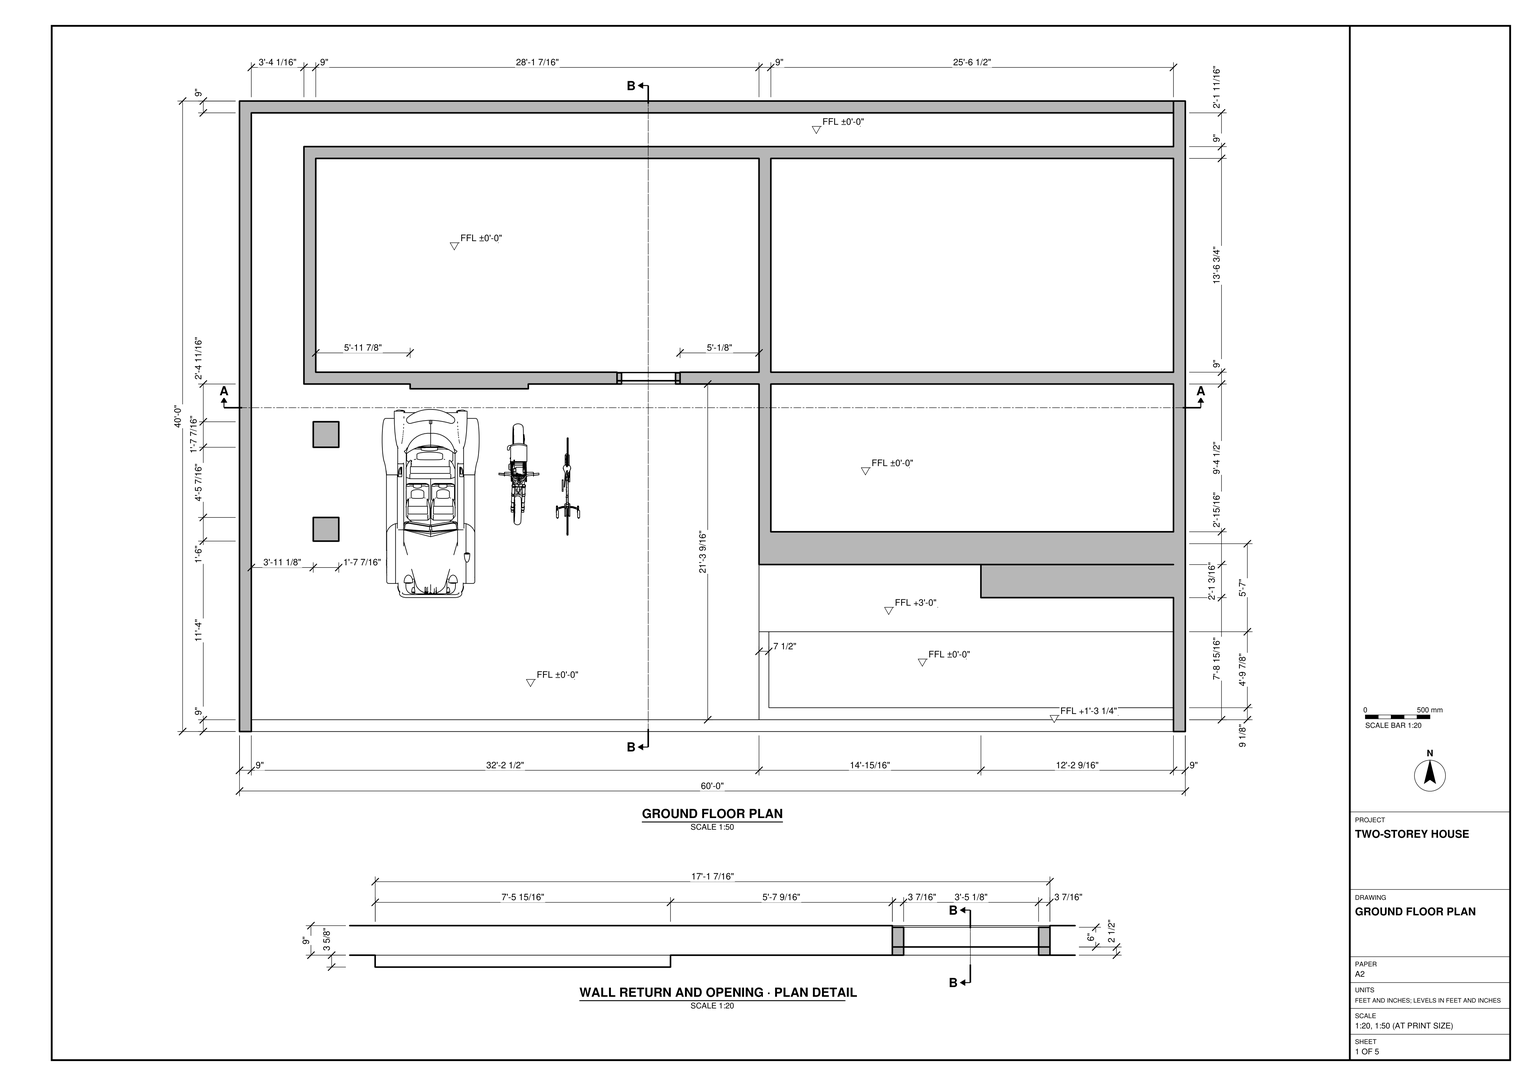
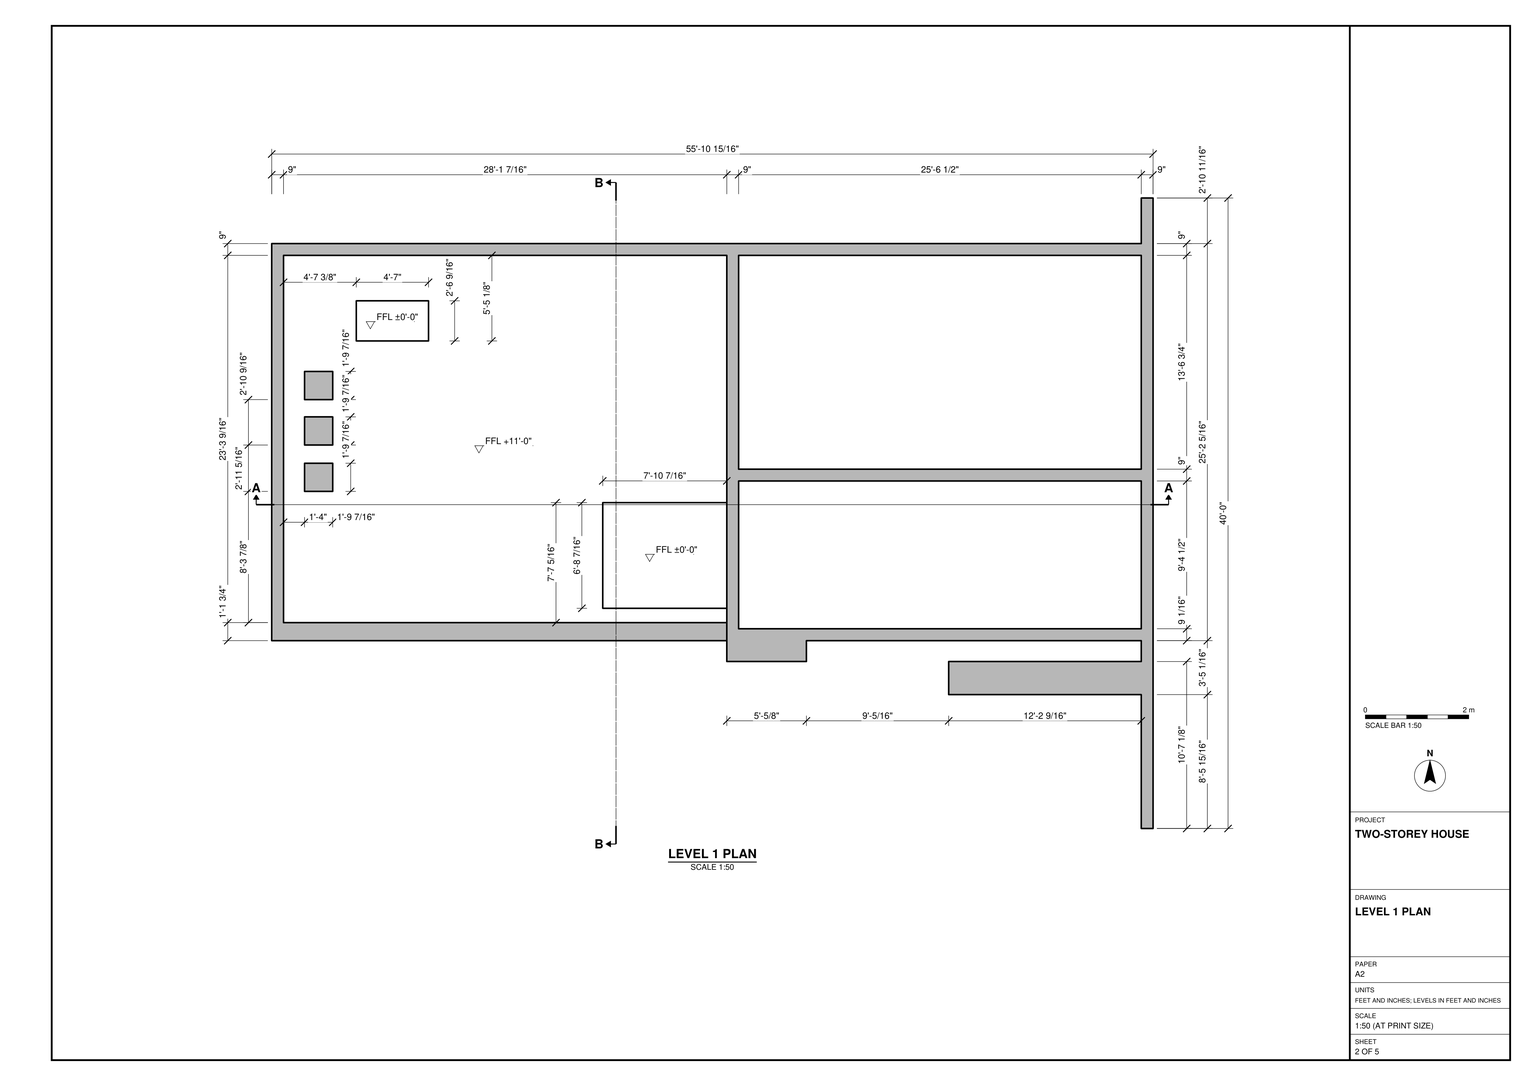
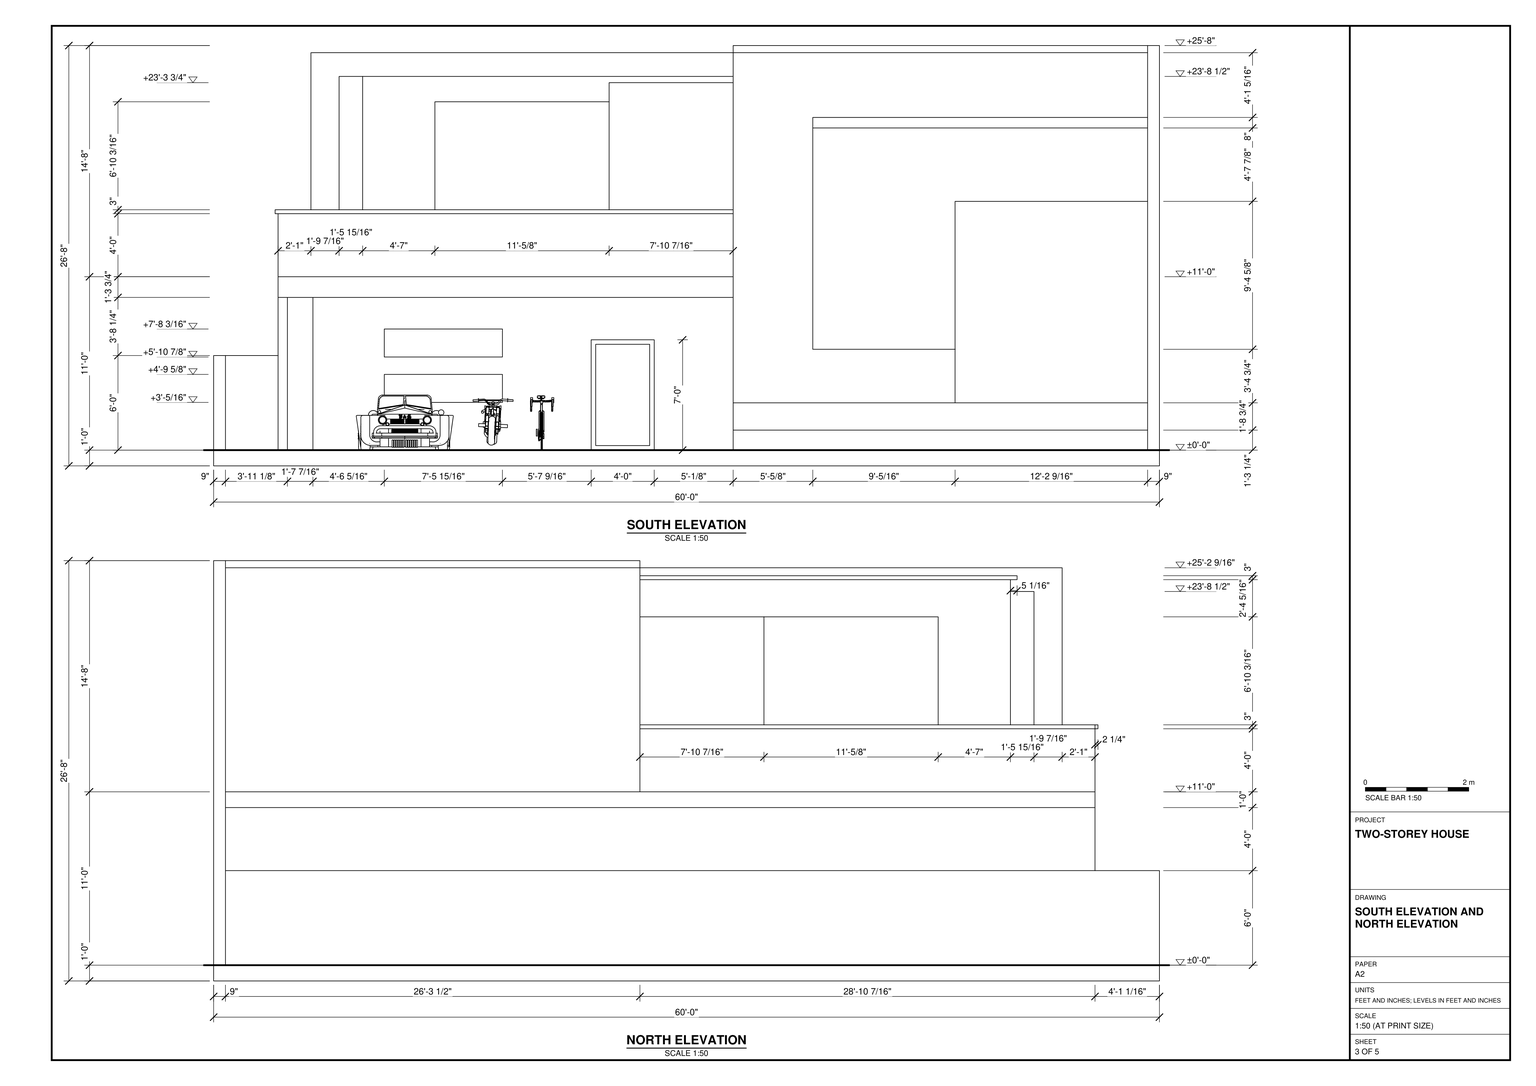
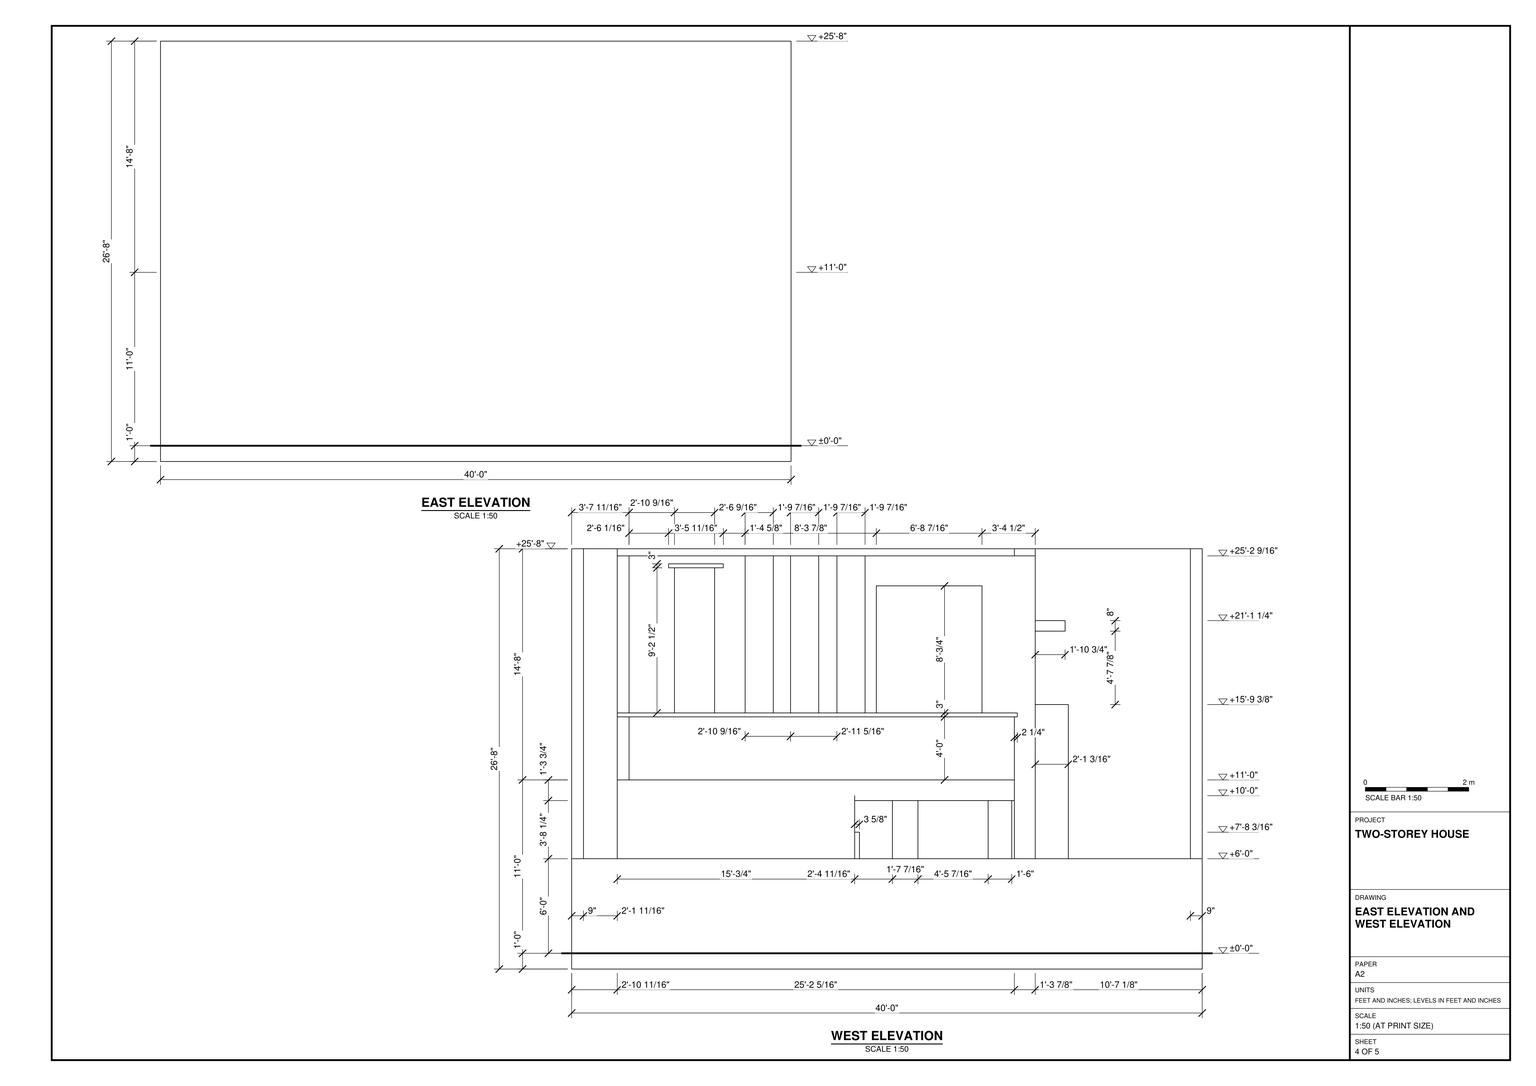
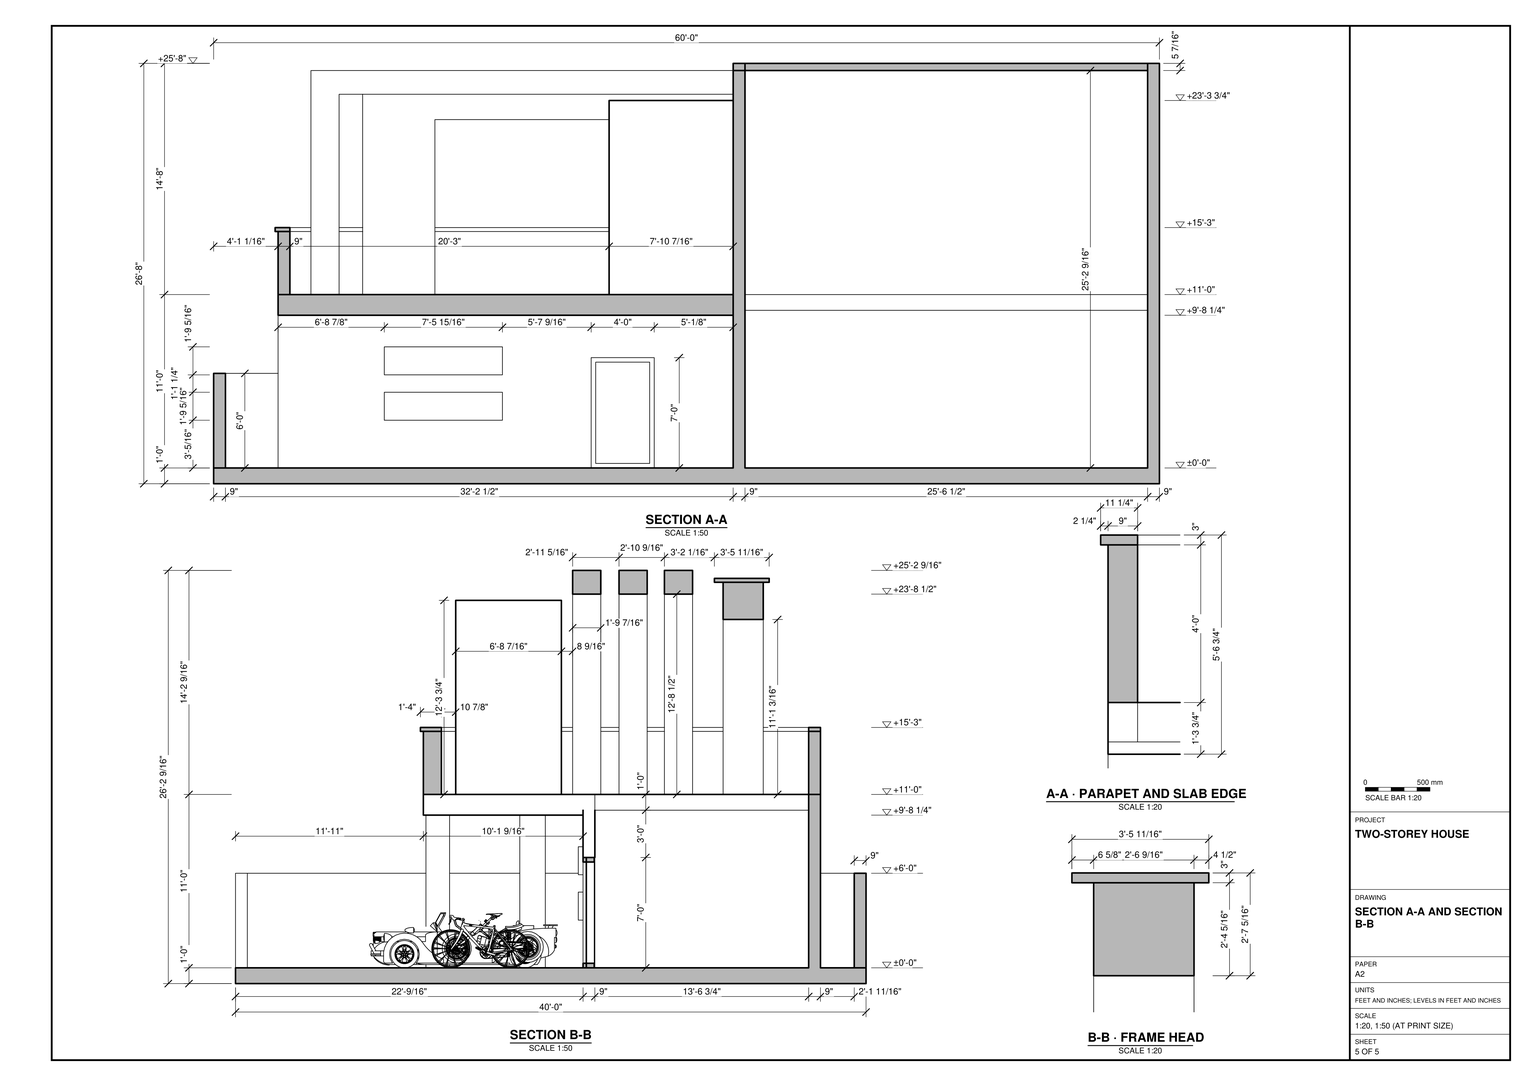
Build the house in SketchUp from task_files/diagram_01.pdf. Work in feet and inches. The overall model is 60'-0" wide from east to west, 40'-0" deep from north to south and 26'-8" high, including the base below the ground floor. Set the ground floor at ±0'-0" and the upper floor at +11'-0".

Use the plans to set out the perimeter walls, the enclosed rear bay and the divided east side of the house. Model the 9" walls with the thicker returns where drawn. Leave the parking bay open to the south, with the upper slab projecting over it and square supports along its west side. Place the car, motorcycle and bicycle as shown. Use the enlarged plan detail for the wall return and framed doorway behind the parking bay, and the south elevation for the window positions.

Carry the central dividing wall through the upper level. Match the slab edges, parapets and flat roof profiles to the elevations, including the tall rectangular frame on the east side of the south facade. Keep walls, slabs and roof elements separate, group each vehicle and any furniture or joinery piece separately, and use components for repeated parts. Decor and loose items may be any suitable library components. Save one SketchUp model as output_files/two_storey_house_with_a_covered_parking_bay.skp.

# SketchUp Ruby script. Lengths in inches.
U = 1.inch
M = Sketchup.active_model
def pt(a) = Geom::Point3d.new(a.map { |v| v * U })
def face(e, loops, mat)
  f = e.add_face(loops[0].map { |a| pt(a) })
  loops[1..].each { |l| e.add_face(l.map { |a| pt(a) }).erase! }
  f.material = f.back_material = mat if mat
  f
end
# faces: each face lists its corners as indices into pts; further lists are holes
def faces(e, pts, list, mat = nil) = list.each { |f| face(e, (f[0].is_a?(Array) ? f : [f]).map { |l| l.map { |i| pts[i] } }, mat) }
# xy, xz, yz: faces in a plane at the given z, y or x. An outline is a flat list of corners, or four numbers for a rectangle; further outlines are holes
def ring(l) = l.size == 4 ? [[l[0], l[1]], [l[2], l[1]], [l[2], l[3]], [l[0], l[3]]] : l.each_slice(2).to_a
def flat(e, list, mat, &to3) = list.each { |f| face(e, (f[0].is_a?(Array) ? f : [f]).map { |l| ring(l).map { |u, v| to3.(u, v) } }, mat) }
def xy(e, z, list, mat = nil) = flat(e, list, mat) { |x, y| [x, y, z] }
def xz(e, y, list, mat = nil) = flat(e, list, mat) { |x, z| [x, y, z] }
def yz(e, x, list, mat = nil) = flat(e, list, mat) { |y, z| [x, y, z] }
def lines(e, pts, list) = list.each { |a, b| e.add_line(pt(pts[a]), pt(pts[b])) }
# prism: a flat outline (further loops are holes) pulled along v
def prism(e, loops, v, mat = nil)
  f = face(e, loops, mat); d = Geom::Vector3d.new(v.map { |x| x * U })
  f.pushpull(f.normal.samedirection?(d) ? d.length : -d.length)
end
def box(e, o, s, mat = nil) = prism(e, [[o, [o[0] + s[0], o[1], o[2]], [o[0] + s[0], o[1] + s[1], o[2]], [o[0], o[1] + s[1], o[2]]]], [0, 0, s[2]], mat)
def at(x, y, z, deg = 0) = Geom::Transformation.translation(pt([x, y, z])) * Geom::Transformation.rotation(ORIGIN, Z_AXIS, deg.degrees)
def axes(o, x, y, z) = Geom::Transformation.new([*x, 0, *y, 0, *z, 0, *pt(o).to_a, 1])
def part(name) = M.definitions.add(name)
# library, detail: a bought-in or finely detailed component or shape, given as its bounding box
def library(name, o, s) = part(name).tap { |d| box(d.entities, o, s) }
def detail(e, o, s) = box(e.add_group.entities, o, s)
def put(e, d, t, mat = nil) = e.add_instance(d, t).tap { |i| i.material = mat if mat }
def group(e, t, mat = nil) = e.add_group.tap { |g| g.transformation = t; g.material = mat if mat }.entities
root = M.entities
M.materials.add("[Blinds Wood Natural]").color = [167, 145, 74]
M.materials.add("[Color B08]").color = [91, 37, 0]
M.materials.add("[Color D01]").color = [255, 242, 204]
M.materials.add("[Color E01]").color = [255, 255, 204]
M.materials.add("[Color M05]").color = [114, 114, 114]
M.materials.add("[Color M06]").color = [86, 86, 86]
M.materials.add("[Color_006]").color = [86, 86, 86]
M.materials.add("[Color_B02]").color = [255, 101, 50]
M.materials.add("[Granite Brown]").color = [126, 104, 91]
M.materials.add("[Grass Dark Green]").color = [106, 157, 55]
M.materials.add("[Metal Seamed]").color = [118, 119, 115]
M.materials.add("[Metal_Aluminum_Anodized]").color = [202, 209, 219]
M.materials.add("[Pavers with Grass Herringbone]").color = [197, 201, 190]
M.materials.add("[Translucent Glass Gray]").color = [128, 128, 128]
M.materials["[Translucent Glass Gray]"].alpha = 0.5
M.materials.add("[Translucent_Glass_Sky_Reflection]").color = [125, 138, 183]
M.materials["[Translucent_Glass_Sky_Reflection]"].alpha = 0.52
M.materials.add("[Wood Veneer 01]").color = [120, 70, 37]
M.materials.add("black1").color = [0, 0, 0]
c1 = library("Car body side",[-13.21,-32.42,-1.14],[59.58,225.6,51.3])
c2 = library("Car fender",[-16.61,0,0],[37.81,73.61,36.77])
c3 = library("Headlamp assembly",[0,0,0],[13.23,21.85,12.42])
c4 = part("Компонент\#2")
xy(c4.entities,0,[[0,2.9375,33.05,6.18]])
xy(c4.entities,23.57,[[4.41,9.77,33.05,11.46]],"[Color_B02]")
yz(c4.entities,0,[[0,0,0,5.92,7.73,19.89,9.03,19.17,1.69,5.92,6.18,0]],"[Color_B02]")
yz(c4.entities,1.28,[[1.01,6.8,6.85,17.36,6.45,17.58,0.61,7.02]],"[Color_006]")
yz(c4.entities,4.41,[[11.0625,22.85,9.77,23.57,11.46,23.57]],"[Color_B02]")
yz(c4.entities,31.57,[[3.7,11.67,3.3,11.89,9.17,22.49,9.5625,22.27]],"[Color_006]")
yz(c4.entities,33.05,[[2.9375,0,6.18,0,2.9375,4.28],[2.9375,4.28,1.69,5.92,2.9375,8.17]])
yz(c4.entities,33.05,[[2.9375,8.17,11.46,23.57,9.77,23.57,2.9375,11.23]],"[Color_006]")
p = [[0,0,0],[33.05,2.9375,11.23],[0,0,5.92],[3.91,0.35,2.11],[3.67,0.33,1.75],[3.34,0.3,1.46],
  [2.94,0.26,1.27],[2.52,0.22,1.1875],[2.08,0.18,1.22],[1.67,0.15,1.36],[1.31,0.12,1.61],[1.02,0.09,1.94],
  [0.83,0.07,2.34],[0.75,0.07,2.77],[0.78,0.07,3.2],[0.93,0.08,3.62],[1.17,0.1,3.98],[1.5,0.13,4.26],
  [1.9,0.17,4.45],[2.32,0.21,4.54],[2.76,0.25,4.5],[3.17,0.28,4.36],[3.53,0.3125,4.11],[3.82,0.34,3.78],
  [4.01,0.36,3.39],[4.09,0.36,2.96],[4.06,0.36,2.52],[0,6.18,0],[0,1.69,5.92],[33.05,1.69,5.92],
  [33.05,2.9375,4.28],[33.05,6.18,0],[3.68,0.14,1.75],[3.93,0.16,2.11],[4.07,0.18,2.52],[4.1,0.18,2.96],
  [4.02,0.17,3.39],[3.83,0.15,3.78],[3.55,0.13,4.11],[3.1875,0.1,4.36],[2.78,0.0625,4.5],[2.34,0.02,4.54],
  [1.91,-0.02,4.45],[1.52,-0.05,4.26],[1.1875,-0.08,3.98],[0.94,-0.1,3.62],[0.8,-0.11,3.2],[0.77,-0.12,2.77],
  [0.85,-0.11,2.34],[1.04,-0.09,1.94],[1.33,-0.07,1.61],[1.6875,-0.04,1.36],[2.1,0,1.22],[2.53,0.04,1.1875],
  [2.96,0.08,1.27],[3.35,0.11,1.46],[0,7.73,19.89],[33.05,9.77,23.57],[4.41,9.77,23.57],[4.21,9.77,23.57],
  [3.7,9.7,23.46],[3.2,9.62,23.3],[2.73,9.51,23.11],[2.28,9.38,22.87],[1.86,9.23,22.6],[1.47,9.06,22.29],
  [1.11,8.87,21.95],[0.8,8.66,21.58],[0.53,8.45,21.18],[0.31,8.22,20.77],[0.13,7.98,20.34],[1.28,0.61,7.02],
  [1.28,6.45,17.58],[1.32,6.77,18.15],[1.42,7.07,18.71],[1.6,7.375,19.25],[1.85,7.66,19.77],[2.17,7.9375,20.27],
  [2.54,8.19,20.73],[2.98,8.43,21.15],[3.46,8.63,21.52],[3.99,8.8125,21.85],[4.56,8.96,22.12],[5.16,9.08,22.33],
  [5.78,9.17,22.49],[31.57,9.17,22.49],[31.57,3.3,11.89],[0,9.03,19.17],[0.13,9.27,19.62],[0.31,9.51,20.05],
  [0.53,9.74,20.47],[0.8,9.96,20.86],[1.11,10.16,21.23],[1.47,10.35,21.57],[1.86,10.52,21.88],[2.28,10.67,22.15],
  [2.73,10.81,22.39],[3.2,10.91,22.59],[3.7,11,22.74],[4.21,11.0625,22.85],[4.41,11.0625,22.85],[4.41,11.46,23.57],
  [33.05,11.46,23.57],[33.05,2.9375,8.17],[31.57,3.7,11.67],[1.28,1.01,6.8],[31.57,9.5625,22.27],[5.78,9.5625,22.27],
  [5.16,9.48,22.11],[4.56,9.36,21.9],[3.99,9.21,21.63],[3.46,9.03,21.3],[2.98,8.82,20.93],[2.54,8.59,20.51],
  [2.17,8.33,20.05],[1.85,8.0625,19.55],[1.6,7.77,19.03],[1.42,7.47,18.49],[1.32,7.16,17.93],[1.28,6.85,17.36]]
faces(c4.entities,p,[[[0,1,2],[3,4,5,6,7,8,9,10,11,12,13,14,15,16,17,18,19,20,21,22,23,24,25,26]],[27,28,29,30,31],[9,8,52,51],[8,7,53,52],[7,6,54,53],[6,5,55,54],[10,9,51,50],[5,4,32,55],
  [11,10,50,49],[4,3,33,32],[12,11,49,48],[3,26,34,33],[13,12,48,47],[26,25,35,34],[14,13,47,46],[25,24,36,35],
  [15,14,46,45],[24,23,37,36],[16,15,45,44],[23,22,38,37],[17,16,44,43],[22,21,39,38],[18,17,43,42],[21,20,40,39],
  [19,18,42,41],[20,19,41,40]],"[Color_B02]")
faces(c4.entities,p,[[32,33,34,35,36,37,38,39,40,41,42,43,44,45,46,47,48,49,50,51,52,53,54,55]],"black1")
faces(c4.entities,p,[[[56,2,1,57,58,59,60,61,62,63,64,65,66,67,68,69,70],[71,72,73,74,75,76,77,78,79,80,81,82,83,84,85,86]],[71,86,104,105],[73,72,119,118],[74,73,118,117],[75,74,117,116],[76,75,116,115],[56,70,88,87],[77,76,115,114],
  [70,69,89,88],[78,77,114,113],[69,68,90,89],[79,78,113,112],[68,67,91,90],[80,79,112,111],[67,66,92,91],[66,65,93,92],
  [81,80,111,110],[82,81,110,109],[65,64,94,93],[83,82,109,108],[64,63,95,94],[84,83,108,107],[63,62,96,95],[85,84,107,106],
  [62,61,97,96],[61,60,98,97],[60,59,99,98],[59,58,100,99]],"[Color_006]")
faces(c4.entities,p,[[28,87,88,89,90,91,92,93,94,95,96,97,98,99,100,101,102,103,29],[106,107,108,109,110,111,112,113,114,115,116,117,118,119,105,104]],"[Translucent_Glass_Sky_Reflection]")
c5 = library("car seat LX",[33.76,-40.52,0],[45.16,29.97,43.35])
c6 = library("V&S",[0.25,0,0],[14.95,5.91,1.01])
c7 = library("Группа\#1",[0,0,0],[18.125,181.43,33.48])
c8 = library("Группа\#13",[0,0,0],[68.98,3.31,14.01])
c9 = part("Компонент\#1")
prism(c9.entities,[[[0,25.02,12.55],[0,25.02,3.45],[0,23.22,3.51],[0,21.43,3.7],[0,19.65,4.03],[0,17.91,4.49],[0,16.21,5.09],[0,14.56,5.8125],[0,12.96,6.66],[0,11.44,7.62],[0,9.99,8.7],[0,8.64,9.89],[0,7.37,11.17],[0,6.21,12.55]]],[1.69,0,0])
c10 = part("Группа\#14")
put(c10.entities,c9,at(0,0,0))
put(c10.entities,c9,at(2.53,0,0))
put(c10.entities,c9,at(5.06,0,0))
put(c10.entities,c9,at(7.58,0,0),"[Color_006]")
put(c10.entities,c9,at(10.11,0,0))
put(c10.entities,c9,at(12.64,0,0))
c11 = library("Группа\#60",[0,0,0],[5.03,11.8,3.54])
c12 = library("Группа\#66",[0,0,0],[12.89,48.17,24.375])
c13 = part("Группа\#69")
prism(c13.entities,[[[0,3.95,0],[0,17.19,0],[2.54,17.19,0],[5.07,17.04,0],[7.59,16.73,0],[10.09,16.27,0],[12.56,15.66,0],[14.98,14.89,0],[17.35,13.99,0],[19.66,12.9375,0],[21.9,11.75,0],[24.07,10.42,0],[26.15,8.97,0],[28.14,7.39,0],[28.8,6.7,0],[29.28,5.88,0],[29.56,4.98,0],[29.63,4.03,0],[29.49,3.09,0],[29.14,2.21,0],[28.6,1.43,0],[27.9,0.79,0],[27.07,0.32,0],[26.16,0.06,0],[25.21,0,0],[24.27,0.16,0],[22.3,0.71,0],[20.31,1.22,0],[18.31,1.69,0],[16.3,2.11,0],[14.28,2.49,0],[12.26,2.83,0],[10.23,3.125,0],[8.1875,3.375,0],[6.15,3.58,0],[4.1,3.75,0],[2.05,3.87,0]]],[0,0,1.14])
c14 = part("Группа\#67")
prism(c14.entities,[[[0,3.95,0],[0,17.19,0],[2.54,17.19,0],[5.07,17.04,0],[7.59,16.73,0],[10.09,16.27,0],[12.56,15.66,0],[14.98,14.89,0],[17.35,13.99,0],[19.66,12.9375,0],[21.9,11.75,0],[24.07,10.42,0],[26.15,8.97,0],[28.14,7.39,0],[28.8,6.7,0],[29.28,5.88,0],[29.56,4.98,0],[29.63,4.03,0],[29.49,3.09,0],[29.14,2.21,0],[28.6,1.43,0],[27.9,0.79,0],[27.07,0.32,0],[26.16,0.06,0],[25.21,0,0],[24.27,0.16,0],[22.3,0.71,0],[20.31,1.22,0],[18.31,1.69,0],[16.3,2.11,0],[14.28,2.49,0],[12.26,2.83,0],[10.23,3.125,0],[8.1875,3.375,0],[6.15,3.58,0],[4.1,3.75,0],[2.05,3.87,0]]],[0,0,1.14])
c15 = part("Группа\#68")
put(c15.entities,c13,axes([29.63,0,0],[-1,0,0],[0,1,0],[0,0,1]))
put(c15.entities,c14,at(29.63,0,0))
c16 = library("Группа\#65",[0,0,0],[10.61,10.21,10.61])
c17 = part("Car")
prism(c17.entities,[[[31.54,107.23,40.23],[31.57,107.31,40.21],[31.63,107.38,40.2],[31.7,107.43,40.19],[31.78,107.47,40.19],[31.87,107.48,40.2],[31.96,107.47,40.21],[32.04,107.44,40.23],[32.11,107.39,40.25],[32.16,107.32,40.27],[32.2,107.25,40.29],[32.21,107.16,40.32],[32.2,107.08,40.34],[32.16,107,40.36],[32.11,106.93,40.37],[32.04,106.87,40.375],[31.96,106.84,40.375],[31.87,106.82,40.37],[31.78,106.83,40.36],[31.7,106.86,40.34],[31.63,106.91,40.32],[31.57,106.98,40.3],[31.54,107.06,40.28],[31.53,107.14,40.25]]],[-0.32,0.84,3.2])
put(c17.entities,c1,at(0.06,94.34,5.18))
put(c17.entities,c1,axes([-26.37,94.34,5.18],[-1,0,0],[0,1,0],[0,0,1]))
put(c17.entities,c2,at(19.89,77.73,5.84))
put(c17.entities,c2,axes([-45.88,77.73,5.84],[-1,0,0],[0,1,0],[0,0,1]))
put(c17.entities,c3,axes([-32.52,66.23,29.86],[-1,0,0],[0,1,0],[0,0,1]))
put(c17.entities,c4,at(-46.77,143.47,44.11,-9.5))
put(c17.entities,c4,axes([20.46,143.59,44.11],[-0.9857,-0.16849,0],[-0.16849,0.9857,0],[0,0,1]))
put(c17.entities,c5,at(-23.08,121.72,9.72,90))
put(c17.entities,c5,at(-54.46,121.72,9.72,90))
put(c17.entities,c5,axes([-65.29,176.97,9.72],[0,0.87005,0],[-2.02657,0,0],[0,0,1.11]))
put(c17.entities,c3,at(6.43,66.23,29.86))
put(c17.entities,c6,axes([-20.66,73.12,37.83],[1,0,0],[0,0,1],[0,-8.245,0]),"[Color_B02]")
put(c17.entities,c7,at(24.36,86.56,0.01))
put(c17.entities,c8,axes([-51.45,67.18,15.21],[1.11,0,0],[0,0.97478,0.53095],[0,-0.53095,0.97478]),"[Metal_Aluminum_Anodized]")
put(c17.entities,c10,at(-11.8125,59.78,0),"[Color_006]")
put(c17.entities,c10,at(-28.8,59.78,0),"[Color_006]")
put(c17.entities,c11,at(22.51,208.75,36.54))
put(c17.entities,c11,axes([-48.51,208.75,36.54],[-1,0,0],[0,1,0],[0,0,1]))
put(c17.entities,c12,at(18.77,242.59,24.34))
put(c17.entities,c12,axes([-44.98,242.59,24.34],[-1,0,0],[0,1,0],[0,0,1]))
put(c17.entities,c15,at(-42.79,274.2,51.77),"[Color_B02]")
put(c17.entities,c7,axes([-52.25,86.56,0.01],[-1,0,0],[0,1,0],[0,0,1]))
put(c17.entities,c16,axes([34.92,115.48,42.84],[-0.6364,0,0],[0,-1.14552,0],[0,0,0.6364]))
c18 = library("Group\#44",[0,-0.05,0],[74.32,17.92,41.45])
c19 = library("Group\#84",[0,-3.47,-3.78],[30.51,80.41,41.33])
xy(root,0,[[0,0,720,480]])
xy(root,12,[[0,0,0,480,711,480,711,471,9,471,9,0],[9,0,711,9],[395.5,9,395.5,76,402.99,76,402.99,18.15,711,18.15,711,9],[56.15,144.97,75.59,162.97],[404.5,152.0625,711,264.5625],
  [56.15,216.41,75.59,235.85],[58.0625,273.5625,395.5,436.3125],[404.5,273.5625,711,436.3125]])
xy(root,12,[[402.99,18.15,711,76]],"[Grass Dark Green]")
xy(root,12,[[[9,9,395.5,9,395.5,264.5625,335.39,264.5625,335.39,273.5625,287.39,273.5625,287.39,264.5625,49.0625,264.5625,49.0625,445.3125,711,445.3125,711,471,9,471],[56.15,216.41,75.59,235.85],[56.15,144.97,75.59,162.97]]],"[Pavers with Grass Herringbone]")
xy(root,27.25,[[395.5,9,711,9,711,18.15,402.99,18.15,402.99,76,395.5,76]])
xy(root,48,[[395.5,127.125,711,143]])
xy(root,48,[[395.5,76,711,76,711,101.93,564.41,101.93,564.41,127.125,395.5,127.125]],"[Grass Dark Green]")
xy(root,48.32,[[129.91,260.9375,219.85,264.5625]],"[Wood Veneer 01]")
xy(root,69.63,[[129.91,260.9375,219.85,264.5625]],"[Wood Veneer 01]")
xy(root,82.88,[[129.91,260.9375,219.85,264.5625]],"[Wood Veneer 01]")
xy(root,84,[[0,0,9,0,9,471,711,471,711,480,0,480]],"[Color E01]")
xy(root,88.77,[[456.1,127.125,711,143]],"[Color D01]")
xy(root,96,[[287.39,264.5625,335.39,273.5625]])
xy(root,104.2,[[129.91,260.9375,219.85,264.5625]],"[Wood Veneer 01]")
xy(root,128.25,[[[49.0625,143,49.0625,264.5625,395.5,264.5625,395.5,143,75.59,143,75.59,162.97,56.15,162.97,56.15,143],[56.15,216.41,75.59,235.85]],[56.15,143,75.59,144.97],[56.15,144.97,75.59,162.97]])
xy(root,144,[[49.0625,143,49.0625,445.3125,395.5,445.3125,395.5,436.3125,58.0625,436.3125,58.0625,156.74,395.5,156.74,395.5,143],[301.0625,167.64,395.5,248.08],[404.5,273.5625,711,436.3125]])
xy(root,144,[[[58.0625,156.74,395.5,156.74,395.5,167.64,301.0625,167.64,301.0625,248.08,395.5,248.08,395.5,436.3125,58.0625,436.3125],[113.4375,371.18,168.4375,401.74],[74.0625,326.51,95.5,347.95],[74.0625,291.95,95.5,313.38],[74.0625,256.63,95.5,278.07]]],"[Granite Brown]")
xy(root,192,[[46.8125,140.75,395.5,143],[46.8125,143,49.0625,445.3125],[49.0625,143,49.0625,445.3125,58.0625,445.3125,58.0625,156.74,395.5,156.74,395.5,143],[58.0625,436.3125,395.5,445.3125]])
xy(root,195,[[46.8125,140.75,395.5,140.75,395.5,156.74,58.0625,156.74,58.0625,436.3125,395.5,436.3125,395.5,445.3125,46.8125,445.3125]],"[Metal Seamed]")
xy(root,201.375,[[564.41,101.93,711,127.125]],"[Blinds Wood Natural]")
xy(root,257.27,[[456.1,104.375,711,143]])
xy(root,265.27,[[456.1,127.125,711,143]])
xy(root,265.27,[[456.1,104.375,711,127.125]],"[Color M06]")
xy(root,277.2,[[168.4375,371.18,395.5,401.74]])
xy(root,291.75,[[301.0625,167.64,395.5,248.08]],"[Blinds Wood Natural]")
xy(root,296.5,[[95.5,256.63,395.5,278.07],[95.5,291.95,395.5,313.38],[95.5,326.51,395.5,347.95]],"[Color M06]")
xy(root,305.5,[[108.375,364.56,395.5,371.18],[108.375,371.18,113.4375,406.24],[113.4375,371.18,395.5,401.74],[113.4375,401.74,395.5,406.24]])
xy(root,308.5,[[108.375,364.56,395.5,406.24]])
xy(root,314.5625,[[395.5,127.125,395.5,445.3125,711,445.3125,711,436.3125,404.5,436.3125,404.5,273.5625,711,273.5625,711,264.5625,404.5,264.5625,404.5,152.0625,711,152.0625,711,127.125],[404.5,152.0625,711,264.5625],[404.5,273.5625,711,436.3125]])
xy(root,314.5625,[[74.0625,256.63,395.5,278.07],[74.0625,291.95,395.5,313.38],[74.0625,326.51,395.5,347.95]],"[Color M06]")
xy(root,320,[[404.5,152.0625,711,264.5625],[404.5,273.5625,711,436.3125]])
xy(root,320,[[711,0,720,480]],"[Color E01]")
xy(root,320,[[395.5,127.125,711,127.125,711,152.0625,404.5,152.0625,404.5,264.5625,711,264.5625,711,273.5625,404.5,273.5625,404.5,436.3125,711,436.3125,711,445.3125,395.5,445.3125]],"[Color M06]")
xz(root,0,[[0,0,720,0,720,320,711,320,711,12,0,12]],"[Color D01]")
xz(root,0,[[0,12,9,84]],"[Color E01]")
xz(root,9,[[395.5,12,711,27.25]],"[Color D01]")
xz(root,18.15,[[402.99,12,711,27.25]])
xz(root,76,[[395.5,12,402.99,27.25]])
xz(root,76,[[402.99,12,711,12,711,48,395.5,48,395.5,27.25,402.99,27.25]],"[Color D01]")
xz(root,101.93,[[564.41,48,711,201.375]],"[Blinds Wood Natural]")
xz(root,104.375,[[456.1,257.27,711,265.27]],"[Color M06]")
xz(root,127.125,[[564.41,48,711,88.77]])
xz(root,127.125,[[564.41,88.77,711,201.375]],"[Blinds Wood Natural]")
xz(root,127.125,[[395.5,48,564.41,48,564.41,88.77,456.1,88.77,456.1,265.27,711,265.27,711,314.5625,395.5,314.5625]],"[Color D01]")
xz(root,127.125,[[395.5,314.5625,711,320]],"[Color M06]")
xz(root,140.75,[[46.8125,192,395.5,195]],"[Metal Seamed]")
xz(root,143,[[456.1,257.27,711,265.27]])
xz(root,143,[[49.0625,128.25,395.5,144]],"[Color D01]")
xz(root,143,[[456.1,88.77,711,257.27],[49.0625,144,395.5,192]],"[Translucent Glass Gray]")
xz(root,144.97,[[56.15,12,75.59,128.25]],"[Color M05]")
xz(root,152.0625,[[404.5,12,711,314.5625],[404.5,314.5625,711,320]])
xz(root,156.74,[[58.0625,192,395.5,195]],"[Metal Seamed]")
xz(root,156.74,[[58.0625,144,395.5,192]],"[Translucent Glass Gray]")
xz(root,162.97,[[56.15,12,75.59,128.25]],"[Color M05]")
xz(root,167.64,[[301.0625,144,395.5,291.75]],"[Blinds Wood Natural]")
xz(root,216.41,[[56.15,12,75.59,128.25]],"[Color M05]")
xz(root,235.85,[[56.15,12,75.59,128.25]],"[Color M05]")
xz(root,248.08,[[301.0625,144,395.5,291.75]],"[Blinds Wood Natural]")
xz(root,256.63,[[74.0625,144,95.5,144,95.5,296.5,395.5,296.5,395.5,314.5625,74.0625,314.5625]],"[Color M06]")
xz(root,260.9375,[[129.91,48.32,219.85,69.63],[129.91,82.88,219.85,104.2]],"[Wood Veneer 01]")
xz(root,264.5625,[[404.5,12,711,132],[49.0625,128.25,395.5,132],[404.5,132,711,144],[404.5,144,711,314.5625],[404.5,314.5625,711,320]])
xz(root,264.5625,[[[49.0625,12,287.39,12,287.39,96,335.39,96,335.39,12,395.5,12,395.5,128.25,49.0625,128.25],[129.91,82.88,219.85,104.2],[129.91,48.32,219.85,69.63]]],"[Color D01]")
xz(root,273.5625,[[58.0625,12,58.0625,132,395.5,132,395.5,12,335.39,12,335.39,96,287.39,96,287.39,12],[404.5,12,711,132],[404.5,132,711,144],[404.5,144,711,314.5625],[404.5,314.5625,711,320]])
xz(root,278.07,[[74.0625,144,74.0625,314.5625,395.5,314.5625,395.5,296.5,95.5,296.5,95.5,144]],"[Color M06]")
xz(root,291.95,[[74.0625,144,95.5,144,95.5,296.5,395.5,296.5,395.5,314.5625,74.0625,314.5625]],"[Color M06]")
xz(root,313.38,[[74.0625,144,74.0625,314.5625,395.5,314.5625,395.5,296.5,95.5,296.5,95.5,144]],"[Color M06]")
xz(root,326.51,[[74.0625,144,95.5,144,95.5,296.5,395.5,296.5,395.5,314.5625,74.0625,314.5625]],"[Color M06]")
xz(root,347.95,[[74.0625,144,74.0625,314.5625,395.5,314.5625,395.5,296.5,95.5,296.5,95.5,144]],"[Color M06]")
xz(root,364.56,[[108.375,305.5,395.5,308.5]])
xz(root,371.18,[[113.4375,144,168.4375,144,168.4375,277.2,395.5,277.2,395.5,305.5,113.4375,305.5]])
xz(root,401.74,[[113.4375,144,113.4375,305.5,395.5,305.5,395.5,277.2,168.4375,277.2,168.4375,144]])
xz(root,406.24,[[108.375,305.5,395.5,308.5]])
xz(root,436.3125,[[58.0625,12,395.5,132],[404.5,12,711,132],[58.0625,132,395.5,144],[404.5,132,711,144],[404.5,144,711,314.5625],
  [404.5,314.5625,711,320]])
xz(root,436.3125,[[58.0625,192,395.5,195]],"[Metal Seamed]")
xz(root,436.3125,[[58.0625,144,395.5,192]],"[Translucent Glass Gray]")
xz(root,445.3125,[[49.0625,12,711,132],[49.0625,132,711,144],[395.5,144,711,314.5625]],"[Color E01]")
xz(root,445.3125,[[395.5,314.5625,711,320]],"[Color M06]")
xz(root,445.3125,[[46.8125,192,49.0625,195],[49.0625,192,395.5,195]],"[Metal Seamed]")
xz(root,445.3125,[[49.0625,144,395.5,192]],"[Translucent Glass Gray]")
xz(root,471,[[9,12,711,84]],"[Color E01]")
xz(root,480,[[0,0,0,12,711,12,711,320,720,320,720,0],[0,12,711,84]],"[Color E01]")
yz(root,0,[[0,0,480,12],[0,12,480,84]],"[Color E01]")
yz(root,9,[[0,12,9,84],[9,12,471,84]],"[Color E01]")
yz(root,46.8125,[[140.75,192,445.3125,195]],"[Metal Seamed]")
yz(root,49.0625,[[264.5625,12,264.5625,128.25,143,128.25,143,144,445.3125,144,445.3125,12]],"[Color D01]")
yz(root,49.0625,[[436.3125,144,445.3125,192]],"[Metal Seamed]")
yz(root,49.0625,[[143,144,436.3125,192]],"[Translucent Glass Gray]")
yz(root,56.15,[[144.97,12,162.97,128.25],[216.41,12,235.85,128.25]],"[Color M05]")
yz(root,58.0625,[[273.5625,12,436.3125,132],[273.5625,132,436.3125,144]])
yz(root,58.0625,[[156.74,192,436.3125,195]],"[Metal Seamed]")
yz(root,58.0625,[[156.74,144,436.3125,192]],"[Translucent Glass Gray]")
yz(root,74.0625,[[256.63,144,278.07,314.5625],[291.95,144,313.38,314.5625],[326.51,144,347.95,314.5625]],"[Color M06]")
yz(root,75.59,[[144.97,12,162.97,128.25],[216.41,12,235.85,128.25]],"[Color M05]")
yz(root,95.5,[[256.63,144,278.07,296.5],[291.95,144,313.38,296.5],[326.51,144,347.95,296.5]],"[Color M06]")
yz(root,108.375,[[364.56,305.5,406.24,308.5]])
yz(root,113.4375,[[371.18,144,401.74,305.5]])
yz(root,129.91,[[260.9375,48.32,264.5625,69.63],[260.9375,82.88,264.5625,104.2]],"[Wood Veneer 01]")
yz(root,168.4375,[[371.18,144,401.74,277.2]])
yz(root,219.85,[[260.9375,48.32,264.5625,69.63],[260.9375,82.88,264.5625,104.2]],"[Wood Veneer 01]")
yz(root,287.39,[[264.5625,12,273.5625,96]])
yz(root,301.0625,[[167.64,144,248.08,291.75]],"[Blinds Wood Natural]")
yz(root,335.39,[[264.5625,12,273.5625,96]])
yz(root,395.5,[[273.5625,12,436.3125,132],[143,128.25,264.5625,132],[143,132,264.5625,144],[273.5625,132,436.3125,144],[143,144,156.74,192],
  [167.64,144,248.08,291.75],[140.75,192,143,195],[143,192,156.74,195],[436.3125,192,445.3125,195],[364.56,305.5,406.24,308.5]])
yz(root,395.5,[[9,12,76,27.25],[76,12,143,48],[143,12,264.5625,128.25],[[127.125,48,127.125,314.5625,256.63,314.5625,256.63,296.5,278.07,296.5,278.07,314.5625,291.95,314.5625,291.95,296.5,313.38,296.5,313.38,314.5625,326.51,314.5625,326.51,296.5,347.95,296.5,347.95,314.5625,436.3125,314.5625,436.3125,144,248.08,144,248.08,291.75,167.64,291.75,167.64,144,156.74,144,156.74,195,140.75,195,140.75,192,143,192,143,48],[371.18,277.2,401.74,277.2,401.74,305.5,406.24,305.5,406.24,308.5,364.56,308.5,364.56,305.5,371.18,305.5]]],"[Color D01]")
yz(root,395.5,[[436.3125,195,445.3125,314.5625]],"[Color E01]")
yz(root,395.5,[[127.125,314.5625,143,320],[143,314.5625,445.3125,320]],"[Color M06]")
yz(root,402.99,[[18.15,12,76,27.25]])
yz(root,404.5,[[152.0625,12,264.5625,132],[273.5625,12,436.3125,132],[152.0625,132,264.5625,144],[273.5625,132,436.3125,144],[152.0625,144,264.5625,314.5625],
  [273.5625,144,436.3125,314.5625],[152.0625,314.5625,249.08,320],[249.08,314.5625,254.89,320],[254.89,314.5625,264.5625,320],[273.5625,314.5625,281.51,320],
  [281.51,314.5625,285.76,320],[285.76,314.5625,436.3125,320]])
yz(root,456.1,[[127.125,257.27,143,265.27]])
yz(root,456.1,[[127.125,88.77,143,257.27]],"[Color D01]")
yz(root,456.1,[[104.375,257.27,127.125,265.27]],"[Color M06]")
yz(root,564.41,[[101.93,48,127.125,201.375]],"[Blinds Wood Natural]")
yz(root,711,[[9,12,18.15,27.25],[152.0625,12,264.5625,144],[273.5625,12,436.3125,144],[471,12,480,84],[152.0625,144,264.5625,314.5625],
  [273.5625,144,436.3125,314.5625],[104.375,257.27,127.125,265.27],[127.125,257.27,143,265.27],[127.125,265.27,143,314.5625],[127.125,314.5625,143,320],
  [143,314.5625,152.0625,320],[152.0625,314.5625,264.5625,320],[264.5625,314.5625,273.5625,320],[273.5625,314.5625,436.3125,320],[436.3125,314.5625,445.3125,320]])
yz(root,711,[[0,12,9,320],[18.15,12,18.15,27.25,9,27.25,9,320,127.125,320,127.125,265.27,104.375,265.27,104.375,257.27,143,257.27,143,88.77,127.125,88.77,127.125,201.375,101.93,201.375,101.93,48,76,48,76,12]],"[Color D01]")
yz(root,711,[[445.3125,12,471,320],[471,84,480,320]],"[Color E01]")
yz(root,720,[[0,0,480,320]],"[Color E01]")
p = [[711,143,48],[711,143,88.77]]
lines(root,p,[[0,1]])
put(root,c17,axes([153.67,64.53,11.99],[0.62,0,0],[0,0.62,0],[0,0,0.62]))
g1 = group(root,at(287.39,264.5625,12))
xy(g1,0,[[0,0,48,2.5],[0,2.5,48,8.5]],"[Color B08]")
xy(g1,3.45,[[3.45,0,44.55,2.5],[3.45,2.5,44.55,8.5]],"[Color B08]")
xy(g1,80.55,[[3.45,0,44.55,2.5],[3.45,2.5,44.55,8.5]],"[Color B08]")
xy(g1,84,[[0,0,48,2.5],[0,2.5,48,8.5]],"[Color B08]")
xz(g1,0,[[[0,0,48,84],[3.45,3.45,44.55,80.55]]],"[Color B08]")
xz(g1,2.5,[[[0,0,48,84],[3.45,3.45,44.55,80.55]]])
xz(g1,2.5,[[3.45,3.45,44.55,80.55]],"[Color B08]")
xz(g1,8.5,[[[0,0,48,84],[3.45,3.45,44.55,80.55]]],"[Color B08]")
yz(g1,0,[[0,0,2.5,84],[2.5,0,8.5,84]],"[Color B08]")
yz(g1,3.45,[[0,3.45,2.5,80.55],[2.5,3.45,8.5,80.55]],"[Color B08]")
yz(g1,44.55,[[0,3.45,2.5,80.55],[2.5,3.45,8.5,80.55]],"[Color B08]")
yz(g1,48,[[0,0,2.5,84],[2.5,0,8.5,84]],"[Color B08]")
put(root,c18,at(241.1,223.7,12,-90))
put(root,c19,at(197.47,157.38,15.78))
